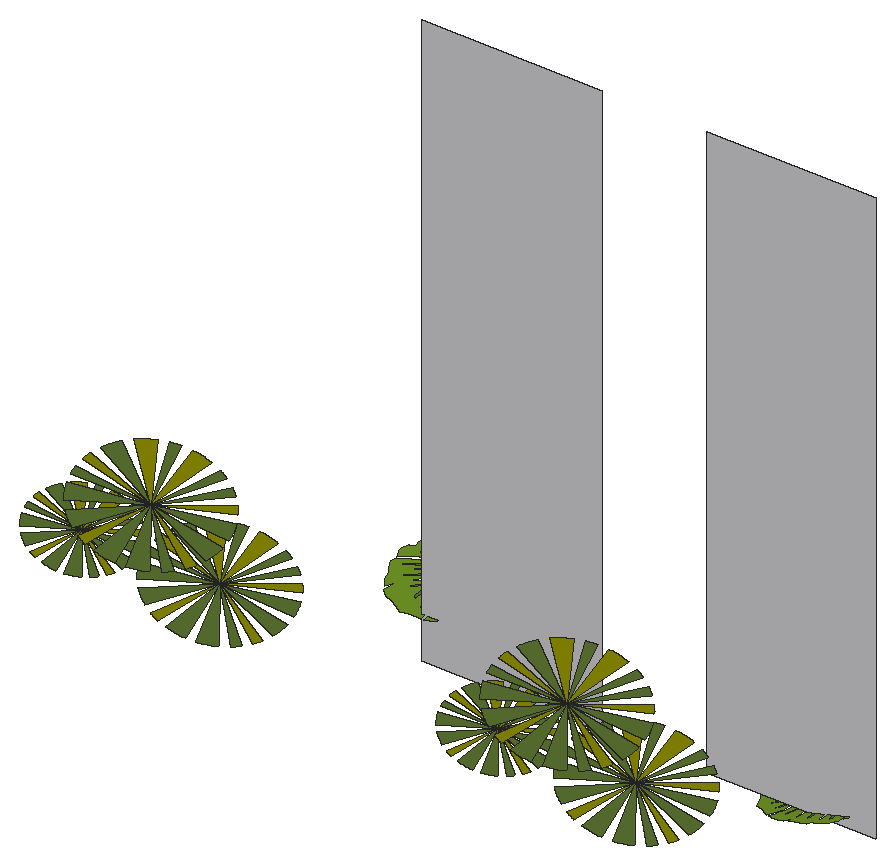
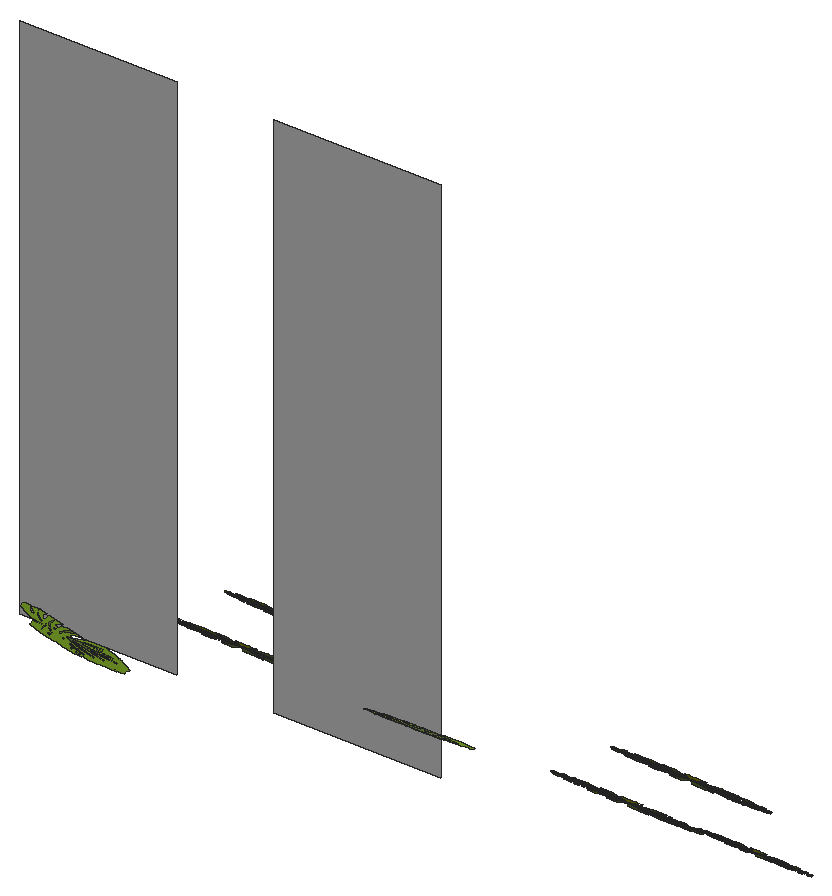
# SketchUp Ruby script. Lengths in inches.
U = 1.inch
M = Sketchup.active_model
def pt(a) = Geom::Point3d.new(a.map { |v| v * U })
def face(e, loops, mat)
  f = e.add_face(loops[0].map { |a| pt(a) })
  loops[1..].each { |l| e.add_face(l.map { |a| pt(a) }).erase! }
  f.material = f.back_material = mat if mat
  f
end
# faces: each face lists its corners as indices into pts; further lists are holes
def faces(e, pts, list, mat = nil) = list.each { |f| face(e, (f[0].is_a?(Array) ? f : [f]).map { |l| l.map { |i| pts[i] } }, mat) }
# xy, xz, yz: faces in a plane at the given z, y or x. An outline is a flat list of corners, or four numbers for a rectangle; further outlines are holes
def ring(l) = l.size == 4 ? [[l[0], l[1]], [l[2], l[1]], [l[2], l[3]], [l[0], l[3]]] : l.each_slice(2).to_a
def flat(e, list, mat, &to3) = list.each { |f| face(e, (f[0].is_a?(Array) ? f : [f]).map { |l| ring(l).map { |u, v| to3.(u, v) } }, mat) }
def xy(e, z, list, mat = nil) = flat(e, list, mat) { |x, y| [x, y, z] }
def xz(e, y, list, mat = nil) = flat(e, list, mat) { |x, z| [x, y, z] }
def yz(e, x, list, mat = nil) = flat(e, list, mat) { |y, z| [x, y, z] }
def lines(e, pts, list) = list.each { |a, b| e.add_line(pt(pts[a]), pt(pts[b])) }
# prism: a flat outline (further loops are holes) pulled along v
def prism(e, loops, v, mat = nil)
  f = face(e, loops, mat); d = Geom::Vector3d.new(v.map { |x| x * U })
  f.pushpull(f.normal.samedirection?(d) ? d.length : -d.length)
end
def box(e, o, s, mat = nil) = prism(e, [[o, [o[0] + s[0], o[1], o[2]], [o[0] + s[0], o[1] + s[1], o[2]], [o[0], o[1] + s[1], o[2]]]], [0, 0, s[2]], mat)
def at(x, y, z, deg = 0) = Geom::Transformation.translation(pt([x, y, z])) * Geom::Transformation.rotation(ORIGIN, Z_AXIS, deg.degrees)
def axes(o, x, y, z) = Geom::Transformation.new([*x, 0, *y, 0, *z, 0, *pt(o).to_a, 1])
def part(name) = M.definitions.add(name)
# library, detail: a bought-in or finely detailed component or shape, given as its bounding box
def library(name, o, s) = part(name).tap { |d| box(d.entities, o, s) }
def detail(e, o, s) = box(e.add_group.entities, o, s)
def put(e, d, t, mat = nil) = e.add_instance(d, t).tap { |i| i.material = mat if mat }
def group(e, t, mat = nil) = e.add_group.tap { |g| g.transformation = t; g.material = mat if mat }.entities
root = M.entities
M.materials.add("[0058_Olive]").color = [128, 128, 0]
M.materials.add("[0059_DarkOliveGreen]").color = [85, 107, 47]
M.materials.add("[0061_OliveDrab]").color = [107, 142, 35]
M.materials.add("[Polished Concrete New]").color = [200, 200, 203]
c1 = part("Group\#77")
p = [[9.84,8.91,4.16],[6.8,0.43,0.2],[7.02,0.37,0.17],[7.24,0.3125,0.15],[7.46,0.26,0.12],[7.68,0.21,0.1],
  [7.91,0.17,0.08],[8.13,0.13,0.0625],[8.36,0.1,0.04],[8.59,0.07,0.03],[8.8125,0.04,0.02],[9.04,0.02,0.01],
  [9.27,0.01,0],[9.5,0,0],[10.87,0.04,0.02],[11.1,0.07,0.03],[11.33,0.1,0.04],[11.55,0.13,0.0625],
  [11.78,0.17,0.08],[12,0.21,0.1],[12.22,0.26,0.12],[12.45,0.3125,0.15],[12.67,0.37,0.17],[12.88,0.43,0.2],
  [13.1,0.5,0.23],[13.32,0.57,0.27],[13.53,0.64,0.3],[4.34,1.52,0.71],[4.43,1.46,0.68],[4.53,1.41,0.66],
  [4.625,1.35,0.63],[4.72,1.3,0.6],[4.82,1.24,0.58],[4.92,1.19,0.55],[5.02,1.14,0.53],[5.12,1.09,0.51],
  [5.22,1.04,0.48],[5.32,0.99,0.46],[5.43,0.94,0.44],[5.53,0.9,0.42],[14.76,1.19,0.55],[14.86,1.24,0.58],
  [14.96,1.3,0.6],[15.06,1.35,0.63],[15.16,1.41,0.66],[15.25,1.46,0.68],[15.35,1.52,0.71],[15.44,1.58,0.74],
  [15.53,1.64,0.76],[15.63,1.7,0.79],[15.72,1.76,0.82],[15.8125,1.82,0.85],[15.9,1.89,0.88],[1.5,4.1875,1.95],
  [1.62,4.01,1.87],[1.75,3.84,1.79],[1.88,3.67,1.71],[2.02,3.51,1.63],[2.16,3.34,1.56],[2.3,3.18,1.48],
  [2.45,3.02,1.41],[2.61,2.87,1.34],[2.76,2.72,1.27],[2.92,2.57,1.2],[3.09,2.43,1.13],[3.26,2.29,1.07],
  [17.81,3.67,1.71],[17.74,3.59,1.67],[17.67,3.51,1.63],[17.6,3.42,1.6],[17.53,3.34,1.56],[17.46,3.26,1.52],
  [17.38,3.18,1.48],[17.31,3.1,1.45],[17.23,3.02,1.41],[17.16,2.95,1.375],[17.08,2.87,1.34],[17,2.79,1.3],
  [16.92,2.72,1.27],[18.53,4.73,2.2],[18.64,4.91,2.29],[18.74,5.1,2.38],[18.83,5.29,2.47],[18.92,5.48,2.55],
  [19.01,5.67,2.64],[19.09,5.86,2.73],[19.17,6.06,2.83],[19.24,6.26,2.92],[19.3,6.46,3.01],[19.36,6.66,3.1],
  [19.42,6.86,3.2],[19.47,7.06,3.29],[0.1,7.67,3.58],[0.13,7.47,3.48],[0.17,7.26,3.39],[0.22,7.06,3.29],
  [0.27,6.86,3.2],[0.32,6.66,3.1],[0.38,6.46,3.01],[0.45,6.26,2.92],[0.52,6.06,2.83],[0.59,5.86,2.73],
  [0.67,5.67,2.64],[0.76,5.48,2.55],[0.85,5.29,2.47],[19.66,8.29,3.87],[19.67,8.5,3.96],[19.68,8.71,4.06],
  [19.69,8.91,4.16],[19.68,9.12,4.25],[19.67,9.33,4.35],[19.66,9.54,4.45],[19.64,9.74,4.54],[19.62,9.95,4.64],
  [19.59,10.16,4.74],[19.55,10.36,4.83],[19.51,10.57,4.93],[19.47,10.77,5.02],[0.1,10.16,4.74],[0.08,10.05,4.6875],
  [0.07,9.95,4.64],[0.05,9.85,4.59],[0.04,9.74,4.54],[0.03,9.64,4.5],[0.02,9.54,4.45],[0.02,9.43,4.4],
  [0.01,9.33,4.35],[0.01,9.23,4.3],[0,9.12,4.25],[0,9.02,4.21],[0,8.91,4.16],[0.85,12.54,5.85],
  [0.8,12.45,5.8],[0.76,12.35,5.76],[0.72,12.26,5.72],[0.67,12.16,5.67],[0.63,12.0625,5.625],[0.59,11.97,5.58],
  [0.56,11.87,5.53],[0.52,11.77,5.49],[0.48,11.67,5.44],[0.45,11.57,5.4],[0.41,11.47,5.35],[0.38,11.375,5.3],
  [3.26,15.54,7.25],[3.09,15.4,7.18],[2.92,15.26,7.12],[2.76,15.11,7.05],[2.61,14.96,6.98],[2.45,14.81,6.9],
  [2.3,14.65,6.83],[2.16,14.49,6.76],[2.02,14.32,6.68],[1.88,14.16,6.6],[1.75,13.99,6.52],[1.62,13.82,6.44],
  [1.5,13.64,6.36],[6.8,17.4,8.11],[6.58,17.33,8.08],[6.37,17.26,8.05],[6.16,17.1875,8.01],[5.94,17.11,7.98],
  [5.73,17.02,7.9375],[5.53,16.93,7.9],[5.32,16.84,7.85],[5.12,16.74,7.81],[4.92,16.64,7.76],[4.72,16.53,7.71],
  [4.53,16.42,7.66],[4.34,16.31,7.61],[9.5,17.83,8.3125],[9.38,17.83,8.3125],[9.27,17.82,8.31],[9.16,17.8125,8.31],
  [9.04,17.81,8.3],[8.93,17.8,8.3],[8.8125,17.79,8.29],[8.7,17.77,8.29],[8.59,17.76,8.28],[8.47,17.75,8.28],
  [8.36,17.73,8.27],[8.25,17.72,8.26],[8.13,17.7,8.25],[19.09,11.97,5.58],[19.05,12.0625,5.625],[19.01,12.16,5.67],
  [18.97,12.26,5.72],[18.92,12.35,5.76],[18.88,12.45,5.8],[18.83,12.54,5.85],[18.79,12.64,5.89],[18.74,12.73,5.9375],
  [18.6875,12.83,5.98],[18.64,12.92,6.02],[18.59,13.01,6.07],[18.53,13.1,6.11],[16.92,15.11,7.05],[17,15.04,7.01],
  [17.08,14.96,6.98],[17.16,14.88,6.94],[17.23,14.81,6.9],[17.31,14.73,6.87],[17.38,14.65,6.83],[17.46,14.57,6.79],
  [17.53,14.49,6.76],[17.6,14.41,6.72],[17.67,14.32,6.68],[17.74,14.24,6.64],[17.81,14.16,6.6],[15.9,15.94,7.43],
  [15.8125,16.01,7.46],[15.72,16.07,7.49],[15.63,16.13,7.52],[15.53,16.19,7.55],[15.44,16.25,7.58],[15.35,16.31,7.61],
  [15.25,16.37,7.63],[15.16,16.42,7.66],[15.06,16.48,7.68],[14.96,16.53,7.71],[14.86,16.59,7.73],[14.76,16.64,7.76],
  [13.53,17.1875,8.01],[13.32,17.26,8.05],[13.1,17.33,8.08],[12.88,17.4,8.11],[12.67,17.46,8.14],[12.45,17.52,8.17],
  [12.22,17.57,8.19],[12,17.62,8.22],[11.78,17.66,8.24],[11.55,17.7,8.25],[11.33,17.73,8.27],[11.1,17.76,8.28],
  [10.87,17.79,8.29]]
faces(c1.entities,p,[[0,1,2,3,4,5,6,7,8,9,10,11,12,13],[0,14,15,16,17,18,19,20,21,22,23,24,25,26],[0,40,41,42,43,44,45,46,47,48,49,50,51,52],[0,53,54,55,56,57,58,59,60,61,62,63,64,65],[0,79,80,81,82,83,84,85,86,87,88,89,90,91],[0,92,93,94,95,96,97,98,99,100,101,102,103,104],[0,105,106,107,108,109,110,111,112,113,114,115,116,117],[0,118,119,120,121,122,123,124,125,126,127,128,129,130],
  [0,144,145,146,147,148,149,150,151,152,153,154,155,156],[0,170,171,172,173,174,175,176,177,178,179,180,181,182],[0,196,197,198,199,200,201,202,203,204,205,206,207,208],[0,209,210,211,212,213,214,215,216,217,218,219,220,221]],"[0059_DarkOliveGreen]")
faces(c1.entities,p,[[0,27,28,29,30,31,32,33,34,35,36,37,38,39],[0,66,67,68,69,70,71,72,73,74,75,76,77,78],[0,131,132,133,134,135,136,137,138,139,140,141,142,143],[0,157,158,159,160,161,162,163,164,165,166,167,168,169],[0,183,184,185,186,187,188,189,190,191,192,193,194,195],[0,222,223,224,225,226,227,228,229,230,231,232,233,234]],"[0058_Olive]")
c2 = part("EXOTIC-AUS-PALM")
put(c2.entities,c1,axes([-13.78,-12.48,-5.82],[1.4,0,0],[0,1.4,0],[0,0,1.4]))
put(c2.entities,c1,at(-21.65,-8.91,-12.03))
put(c2.entities,c1,axes([-1.28,-11.86,-13.4],[1.33,0,0],[0,1.33,0],[0,0,1.33]))
xz(root,148.8,[[408.3,7.8125,454.65,155.375],[481.51,7.8125,525.01,155.375]],"[Polished Concrete New]")
p = [[505.7,160.08,12.43],[503.8,160.49,12.125],[502.07,160.25,11.57],[501.09,159.81,11.12],[500.23,158.99,10.53],[499.84,158.72,10.31],
  [501.92,158.66,10.82],[504.05,158.29,11.2],[506.1,157.7,11.47],[507.58,156.98,11.53],[507.86,156.76,11.49],[507.75,156.68,11.43],
  [507.24,156.77,11.34],[504.82,157.5,11.05],[502.68,157.99,10.71],[500.38,158.38,10.3],[499.15,158.5,10.04],[498.1,158.32,9.69],
  [497.52,157.91,9.35],[496.9,157.24,8.89],[496.39,156.61,8.48],[496.13,156.29,8.27],[495.17,155.76,7.78],[494.5,155.14,7.33],
  [494.09,154.52,6.95],[493.83,154.18,6.73],[494.98,154.23,7.05],[496.74,154.29,7.53],[493.61,153.66,6.44],[493.23,153.48,6.26],
  [493.125,152.9,5.97],[493.02,152.3125,5.68],[493.82,150.98,5.29],[494.22,149.08,4.54],[496.15,148.32,4.7],[497.51,147.55,4.7],
  [498.27,147.06,4.67],[500.25,148.01,5.61],[501.33,148.76,6.23],[502.08,149.83,6.9],[502.55,150.58,7.36],[503.08,150.95,7.66],
  [503.51,151.25,7.91],[503.81,151.25,7.98],[503.9,151.05,7.91],[503.68,150.45,7.59],[503.29,149.95,7.27],[502.09,148.91,6.49],
  [500.99,148.04,5.82],[500.39,147.49,5.41],[499.68,147.13,5.07],[498.93,146.86,4.76],[500.1,146.47,4.88],[501.1,146.29,5.06],
  [501.99,146.1875,5.24],[502.7,146.14,5.41],[503.54,146.04,5.58],[505.08,146.9,6.35],[505.9,147.71,6.93],[506.28,148.42,7.35],
  [506.71,149.74,8.05],[506.83,150.75,8.54],[507.02,151.6,8.97],[507.27,152.24,9.32],[507.71,152.54,9.5625],[508.3,152.56,9.72],
  [508.55,152.08,9.58],[508.71,151.43,9.32],[508.41,150.28,8.73],[507.67,149.05,7.99],[506.49,147.6875,7.07],[504.69,146.15,5.92],
  [507.69,145.98,6.62],[509.47,145.95,7.0625],[510.25,146.2,7.37],[511.07,146.76,7.83],[511.54,147.45,8.26],[511.72,148.38,8.73],
  [511.85,149.17,9.12],[512.01,150.34,9.68],[511.91,151.2,10.05],[511.82,151.88,10.33],[511.7,152.21,10.44],[511.98,152.4,10.6],
  [512.4,152.2,10.62],[512.92,151.7,10.53],[513.18,150.91,10.24],[512.96,149.32,9.47],[512.63,148.39,8.97],[512.18,147.56,8.48],
  [511.76,147.17,8.2],[511.07,146.41,7.68],[511.57,146.38,7.79],[513.29,146.57,8.32],[514.83,146.77,8.81],[516.58,147.54,9.6],
  [516.91,148.35,10.05],[516.66,149.65,10.57],[515.93,150.79,10.89],[515.4,151.83,11.22],[515.13,152.28,11.36],[515.18,152.54,11.49],
  [515.49,152.51,11.55],[516.15,151.98,11.49],[517.06,150.71,11.15],[517.32,149.68,10.75],[517.3125,148.02,10.01],[519.38,148.85,10.92],
  [520.47,149.69,11.57],[520.65,150.4,11.93],[520.3,150.76,12.01],[519.15,151.85,12.2],[518.1,152.66,12.29],[517.43,153.3,12.41],
  [517.35,153.56,12.5],[517.64,153.64,12.61],[517.93,153.5,12.625],[519.32,152.48,12.53],[520.12,151.66,12.36],[520.64,150.93,12.17],
  [520.99,150.375,12.01],[521.75,151.06,12.51],[521.98,151.69,12.86],[521.66,152.51,13.14],[520.98,153.28,13.3125],[520.52,154.07,13.54],
  [519.68,154.47,13.51],[518.65,155.15,13.55],[517.46,155.73,13.51],[515.88,156.01,13.22],[514.24,155.93,12.76],[513.28,155.73,12.43],
  [512.93,156.12,12.52],[513.72,156.45,12.87],[514.53,157.01,13.33],[514.47,157.74,13.64],[513.87,158.8,13.96],[513.27,159.77,14.24],
  [513.01,160.45,14.48],[509.56,160.87,13.78],[507.49,160.84,13.23],[506.28,160.49,12.77],[500.5,157.36,9.87],[504.98,156.86,10.8],
  [507.95,156.01,11.18],[510.48,155.08,11.41],[511.21,155.33,11.72],[510.2,156.27,11.88],[508.87,157.52,12.1],[505.84,158.78,11.88],
  [508.56,157.92,12.2],[510.59,156.93,12.28],[511.375,155.82,11.98],[511.75,155.64,11.99],[512.27,156,12.29],[511.22,157.76,12.8125],
  [510.75,159.75,13.58],[512.82,155.8,12.34],[514.04,155.47,12.51],[516.65,154.95,12.95],[518.29,154.28,13.07],[519.24,153.6875,13.05],
  [516.5,154.6,12.75],[514.23,155.14,12.41],[512.97,155.3,12.16],[514.99,154.55,12.34],[516.9,153.08,12.17],[517.91,151.9,11.9],
  [518.69,150.68,11.56],[518.93,150.07,11.34],[517.35,151.95,11.78],[516.23,153.07,12],[514.72,154.3,12.16],[513.4,154.94,12.11],
  [512.66,155.2,12.04],[512.2,155.14,11.89],[512.1,154.9375,11.77],[512.55,154.39,11.64],[513.26,153.85,11.58],[513.73,153.2,11.41],
  [514.64,151.33,10.8],[514.93,150.13,10.34],[514.66,149.01,9.77],[514.49,148.1,9.32],[513.99,147.76,9.03],[514.35,149.51,9.91],
  [514.24,150.5,10.33],[513.72,152.0625,10.9],[512.87,153.45,11.3],[511.6875,154.96,11.67],[509.83,154.17,10.84],[510.27,153,10.43],
  [510.64,151.9,10.03],[510.29,149.62,8.92],[509.63,148.49,8.24],[509.0625,147.74,7.76],[508.55,147.38,7.47],[509.16,148.45,8.1],
  [509.71,150.21,9.04],[509.88,152.47,10.09],[509.32,153.82,10.55],[505.75,152.61,9.09],[506.02,151.7,8.75],[505.65,150.59,8.16],
  [504.87,149.53,7.48],[504.02,148.72,6.9],[502.75,147.84,6.18],[504.55,149.67,7.46],[505.28,150.72,8.125],[505.52,151.71,8.63],
  [505.34,152.6,8.98],[502.56,151.83,7.92],[502.06,150.85,7.35],[501.19,149.98,6.74],[500.16,149.26,6.15],[499.15,148.95,5.75],
  [500.88,150.15,6.73],[501.57,151.05,7.3125],[501.98,151.77,7.74],[499.82,151.02,6.85],[498.66,150.64,6.38],[497.19,150.08,5.75],
  [497.38,150.18,5.85],[499.55,151.26,6.89],[501.76,152.11,7.84],[504.4,152.76,8.8125],[498.17,153.2,7.41],[505.27,153.2,9.23],
  [507.39,153.97,10.12],[504.33,154.66,9.65],[499.39,155.375,8.7],[503.03,155.12,9.52],[506.39,154.6,10.15],[508.16,154.17,10.41],
  [509.93,154.92,11.21],[506.09,156.15,10.77],[503.34,156.15,10.06],[505.4,155.73,10.4],[505.91,155.51,10.43],[506.02,155.36,10.39],
  [505.79,155.29,10.31],[504.96,155.42,10.15],[503,155.72,9.78],[500.83,156.05,9.37],[498.55,156.3,8.9],[497.48,156.4375,8.68],
  [500.72,156.4,9.5],[503.59,154.21,9.25],[504.32,154.01,9.35],[504.37,153.78,9.26],[504.04,153.66,9.12],[503.32,153.64,8.93],
  [502.75,153.72,8.82],[500.46,154.01,8.36],[498.34,154.29,7.9375],[501.59,154.33,8.79],[507.78,159.47,12.69],[508.76,159.13,12.79],
  [509.67,158.57,12.78],[510.1875,158.08,12.6875],[510.14,157.82,12.56],[509.9,157.73,12.46],[508.35,158.55,12.43],[507.13,159.28,12.44],
  [506.9,159.49,12.48],[511.28,153.26,10.81],[510.86,153.67,10.88],[510.96,154.16,11.125],[511.41,154.3125,11.3125],[511.86,153.98,11.28],
  [511.94,153.55,11.11],[511.67,153.24,10.89],[513.39,154.71,12],[513.71,154.27,11.88],[513.72,153.94,11.74],[513.33,153.96,11.65],
  [512.99,154.43,11.77],[512.96,154.78,11.92],[408.06,160.19,25.91],[408.79,160.06,25.83],[409.23,160.58,26.16],[410.29,161.31,26.62],
  [411.75,161.76,26.9],[413.3,161.83,26.95],[414.86,161.76,26.91],[415.96,161.82,26.94],[417.25,161.45,26.71],[418.68,161.18,26.54],
  [419.92,160.73,26.25],[420.54,160.1875,25.91],[420.84,159.4,25.41],[419.91,159.65,25.56],[418.64,159.95,25.76],[417.07,160.21,25.92],
  [414.83,160.36,26.02],[414.46,160.35,26.01],[414.35,160.17,25.9],[414.72,160.02,25.8],[415.98,159.84,25.69],[417.72,159.7,25.6],
  [419.88,159.39,25.4],[420.58,159.28,25.33],[421.32,158.71,24.97],[421.58,157.67,24.3125],[421.14,156.24,23.41],[419.11,157.42,24.15],
  [417.65,158.04,24.54],[415.43,158.57,24.88],[414.32,158.68,24.95],[414.07,158.57,24.88],[414.35,158.37,24.76],[415.1,158.16,24.62],
  [416.76,157.64,24.29],[418.68,157.13,23.97],[420.45,156.3125,23.45],[421.22,155.61,23],[420.9375,154.35,22.2],[420.1,153.58,21.72],
  [419.11,152.75,21.1875],[418.72,152.57,21.07],[418.29,152.82,21.23],[418.27,153.39,21.59],[418.09,153.83,21.875],[417.38,154.6,22.36],
  [416.46,155.4,22.87],[414.66,156.61,23.64],[413.51,157.0625,23.92],[412.52,157.2,24.01],[411.97,157.18,24],[412.01,156.93,23.84],
  [412.5,156.74,23.72],[413.4,156.3,23.44],[414.54,155.73,23.08],[415.87,154.84,22.51],[416.75,154.23,22.125],[417.77,153.49,21.66],
  [418.4,152.09,20.77],[418.15,151.6,20.46],[416.87,150.9,20.01],[414.53,149.8,19.32],[413.91,151.62,20.47],[413.06,153.06,21.38],
  [412.0625,154.23,22.13],[410.86,155.16,22.72],[409.95,155.5625,22.97],[409.18,155.8,23.12],[408.78,155.54,22.96],[408.84,155.15,22.71],
  [409.45,154.6,22.36],[410.37,153.92,21.93],[411.53,153.16,21.45],[412.86,152.05,20.74],[413.46,151.39,20.33],[413.88,150.48,19.75],
  [413.84,149.26,18.97],[413.13,148.99,18.8],[412.57,148.73,18.64],[411.82,148.4375,18.45],[410.89,148.16,18.28],[409.57,147.97,18.15],
  [409.78,148.46,18.47],[409.83,149,18.81],[409.58,149.64,19.21],[409.28,150.7,19.89],[408.86,151.92,20.66],[408.5,152.43,20.99],
  [407.93,152.94,21.3125],[407.61,153.05,21.375],[407.4,152.93,21.3],[407.47,152.54,21.06],[407.55,152.07,20.75],[408.15,151.34,20.3],
  [408.93,150.28,19.62],[409.09,149.32,19.01],[408.87,147.84,18.07],[407.72,147.88,18.1],[405.82,147.87,18.09],[403.51,147.625,17.9375],
  [400.89,148.81,18.6875],[398.67,149.43,19.08],[398.03,149.88,19.37],[397.39,150.34,19.66],[397.43,150.61,19.83],[398.87,152.33,20.92],
  [397.7,151.58,20.44],[396.94,151.07,20.125],[396.72,151.42,20.34],[396.23,152.03,20.73],[395.95,152.73,21.18],[395.97,153.5,21.66],
  [395.76,153.83,21.875],[395.35,154.48,22.29],[394.95,155.21,22.75],[394.86,155.73,23.08],[395.38,156.29,23.43],[396.4,156.7,23.7],
  [398.52,157.36,24.11],[400.62,157.88,24.45],[403.24,158.34,24.74],[403.71,158.48,24.83],[403.69,158.58,24.89],[403.21,158.63,24.92],
  [401.28,158.54,24.86],[399.11,158.125,24.6],[397.14,157.52,24.22],[395.61,156.72,23.71],[395.55,157.07,23.93],[395.14,158,24.52],
  [395.29,158.7,24.97],[396.22,159.58,25.52],[398.06,160.0625,25.83],[397.97,160.59,26.16],[398.39,161.32,26.63],[399.83,162.18,27.17],
  [402.78,163.29,27.875],[403.8,162.91,27.63],[405.42,162.46,27.35],[407.15,161.96,27.03],[408.09,161.47,26.72],[408.21,160.75,26.26],
  [406.25,155.02,22.625],[401.22,152.14,20.8],[406.17,154.36,22.21],[405.1,152.83,21.24],[404.6,151.33,20.28],[404.39,149.69,19.24],
  [404.38,149.54,19.15],[404.73,150.53,19.78],[405.07,151.27,20.25],[405.68,152.67,21.14],[406.29,152,20.71],[406.91,151.08,20.13],
  [407.16,149.53,19.14],[407.48,150.16,19.55],[407.33,151.09,20.13],[406.87,152.06,20.75],[406.01,152.95,21.32],[407.03,154.62,22.375],
  [408.26,154.07,22.02],[409.31,153.27,21.52],[410.09,152.23,20.86],[411.07,150.21,19.57],[410.88,151.35,20.3],[410.49,152.26,20.875],
  [409.73,153.33,21.56],[408.62,154.26,22.15],[407.3125,154.8,22.49],[408.34,157.1,23.95],[410.41,156.37,23.49],[413.07,154.71,22.43],
  [414.85,153.24,21.5],[415.74,152.24,20.86],[415.66,152.69,21.15],[415.14,153.46,21.64],[414.2,154.52,22.3125],[411.64,156.28,23.43],
  [410.03,156.91,23.83],[408.27,157.55,24.24],[408.61,158.87,25.07],[411.3125,158.28,24.69],[413.625,157.65,24.3],[415.92,156.75,23.73],
  [417.22,156.09,23.31],[419.125,154.71,22.43],[419.05,155.15,22.71],[418.05,155.87,23.17],[416.86,156.77,23.74],[415.18,157.5,24.2],
  [412.23,158.45,24.81],[411.1,158.72,24.97],[409.92,158.8125,25.04],[408.93,159.02,25.17],[408.75,159.21,25.28],[409,159.4375,25.43],
  [409.85,159.55,25.5],[411.57,159.63,25.55],[414.15,159.375,25.39],[416.32,159.04,25.18],[419.76,158.35,24.74],[418.84,158.68,24.95],
  [416.79,159.22,25.3],[414.62,159.65,25.57],[411.45,159.92,25.74],[409.09,159.63,25.55],[410.2,160.02,25.8],[412.46,160.5625,26.15],
  [415.52,161.03,26.44],[414.125,161.0625,26.46],[412.13,160.88,26.35],[409.65,160.18,25.91],[408.38,159.92,25.74],[402.04,161.875,26.98],
  [404.83,160.66,26.21],[407.74,159.84,25.6875],[407.82,159.37,25.39],[407.33,159.35,25.375],[405.4,159.82,25.67],[402.75,159.69,25.59],
  [399.77,159.19,25.28],[403.46,159.53,25.49],[405.95,159.1875,25.27],[407.82,158.93,25.11],[407.61,158.46,24.8125],[404.67,158.1,24.58],
  [401.53,157.49,24.2],[397.75,156.02,23.27],[403.19,157.4375,24.16],[407.41,158.13,24.6],[407.1,156.88,23.81],[405.32,156.46,23.54],
  [402.3,155.47,22.91],[399.41,154.18,22.09],[403.78,155.68,23.04],[406.8,156.42,23.52],[401.25,156.32,23.45],[399.86,155.75,23.09],
  [399.09,155.4375,22.89],[396.75,154.15,22.08],[397.67,154.49,22.29],[399.59,155.24,22.77],[401.53,155.88,23.18],[403.29,156.46,23.55],
  [404.03,156.71,23.7],[404.12,156.85,23.79],[403.84,156.91,23.83],[403.22,156.86,23.8],[403.03,154.6875,22.42],[402.63,154.5,22.3],
  [402.24,154.33,22.1875],[400,152.98,21.33],[401.84,153.64,21.75],[403.82,154.36,22.21],[404.32,154.54,22.32],[404.81,154.85,22.52],
  [404.89,155.07,22.66],[404.58,155.21,22.75],[403.81,155.05,22.65],[402.07,160.62,26.18],[401.4,160.63,26.1875],[400.28,160.47,26.09],
  [399.64,160.13,25.87],[400.0625,160.07,25.84],[401.82,160.05,25.82],[403.93,160.1,25.85],[404,160.26,25.95],[403.7,160.46,26.08],
  [402.73,160.6,26.17],[409.08,158,24.52],[409.62,157.62,24.28],[410.41,157.5,24.2],[410.72,157.64,24.29],[410.53,157.97,24.5],
  [409.95,158.24,24.67],[409.22,158.3,24.71],[410.67,159.25,25.3125],[410.13,159.38,25.39],[409.73,159.25,25.3125],[410.1875,159.02,25.17],
  [411.01,158.82,25.04],[411.3,158.97,25.14],[410.89,159.2,25.28]]
faces(root,p,[[[0,1,2,3,4,5,6,7,8,9,10,11,12,13,14,15,16,17,18,19,20,21,22,23,24,25,26,27,28,29,30,31,32,33,34,35,36,37,38,39,40,41,42,43,44,45,46,47,48,49,50,51,52,53,54,55,56,57,58,59,60,61,62,63,64,65,66,67,68,69,70,71,72,73,74,75,76,77,78,79,80,81,82,83,84,85,86,87,88,89,90,75,91,92,93,94,95,96,97,98,99,100,101,102,103,104,105,106,107,108,109,110,111,112,113,114,115,116,117,118,119,120,121,122,123,124,125,126,127,128,129,130,131,132,133,134,135,136,137,138,139,140,141],[142,143,144,145,146,147,148,149,150,151,152,153,154,155,156,157,158,159,160,161,162,163,164,165,166,167,168,169,170,171,172,173,174,175,176,177,178,179,180,181,182,183,184,185,186,187,188,189,190,191,192,193,194,195,196,197,198,199,200,201,202,203,204,205,206,207,208,209,210,211,212,213,214,215,216,217,218,219,220,221,222,223,224,225,226,227,228,229,230,231,232,233,234,235],[236,237,238,239,240,241,242,243,244,245,246],[247,248,249,250,251,252,253,254,255],[256,257,258,259,260,261,262,263,264],[265,266,267,268,269,270,271],[272,273,274,275,276,277]],[[278,279,280,281,282,283,284,285,286,287,288,289,290,291,292,293,294,295,296,297,298,299,300,301,302,303,304,305,306,307,308,309,310,311,312,313,314,315,316,317,318,319,320,321,322,323,324,325,326,327,328,329,330,331,332,333,334,335,320,336,337,338,339,340,341,342,343,344,345,346,347,348,349,350,351,352,353,354,355,356,357,358,359,360,361,362,363,364,365,366,367,368,369,370,371,372,373,374,375,376,377,378,379,380,381,382,383,384,385,386,387,388,389,390,391,392,393,394,395,396,397,398,399,400,401,402,403,404,405,406,407,408,409,410,411,412,413,414,415,416,417,418,419],[420,421,422,423,424,425,426,427,428,429,430,431,432,433,434,435,436,437,438,439,440,441,442,443,444,445,446,447,448,449,450,451,452,453,454,455,456,457,458,459,460,461,462,463,464,465,466,467,468,469,470,471,472,473,474,475,476,477,478,479,480,481,482,483,484,485,486,487,488,489,490,491,492,493,494,495,496,497,498,499,500,501,502,503,504,505,506,507,508,509,510,511,512,513],[514,515,516,517,518,519,520,521,522,523,524,525],[526,527,528,529,530,531,532,533,534,535,536],[537,538,539,540,541,542,543,544,545,546],[547,548,549,550,551,552,553],[554,555,556,557,558,559,560]]],"[0061_OliveDrab]")
faces(root,p,[[143,142,235,234,233,232,231,230,229,228,227,226,225,224,223,222,221,220,219,218,217,216,215,214,213,212,211,210,209,208,207,206,205,204,203,202,201,200,199,198,197,196,195,194,193,192,191,190,189,188,187,186,185,184,183,182,181,180,179,178,177,176,175,174,173,172,171,170,169,168,167,166,165,164,163,162,161,160,159,158,157,156,155,154,153,152,151,150,149,148,147,146,145,144],[421,420,513,512,511,510,509,508,507,506,505,504,503,502,501,500,499,498,497,496,495,494,493,492,491,490,489,488,487,486,485,484,483,482,481,480,479,478,477,476,475,474,473,472,471,470,469,468,467,466,465,464,463,462,461,460,459,458,457,456,455,454,453,452,451,450,449,448,447,446,445,444,443,442,441,440,439,438,437,436,435,434,433,432,431,430,429,428,427,426,425,424,423,422]],"[0059_DarkOliveGreen]")
put(root,c2,axes([345.71,140,25.5],[1.5,0,0],[0,0.86025,0],[0,0,1.5]))
put(root,c2,axes([457.9,133.53,21.92],[1.5,0,0],[0,0.86025,0],[0,0,1.5]))
